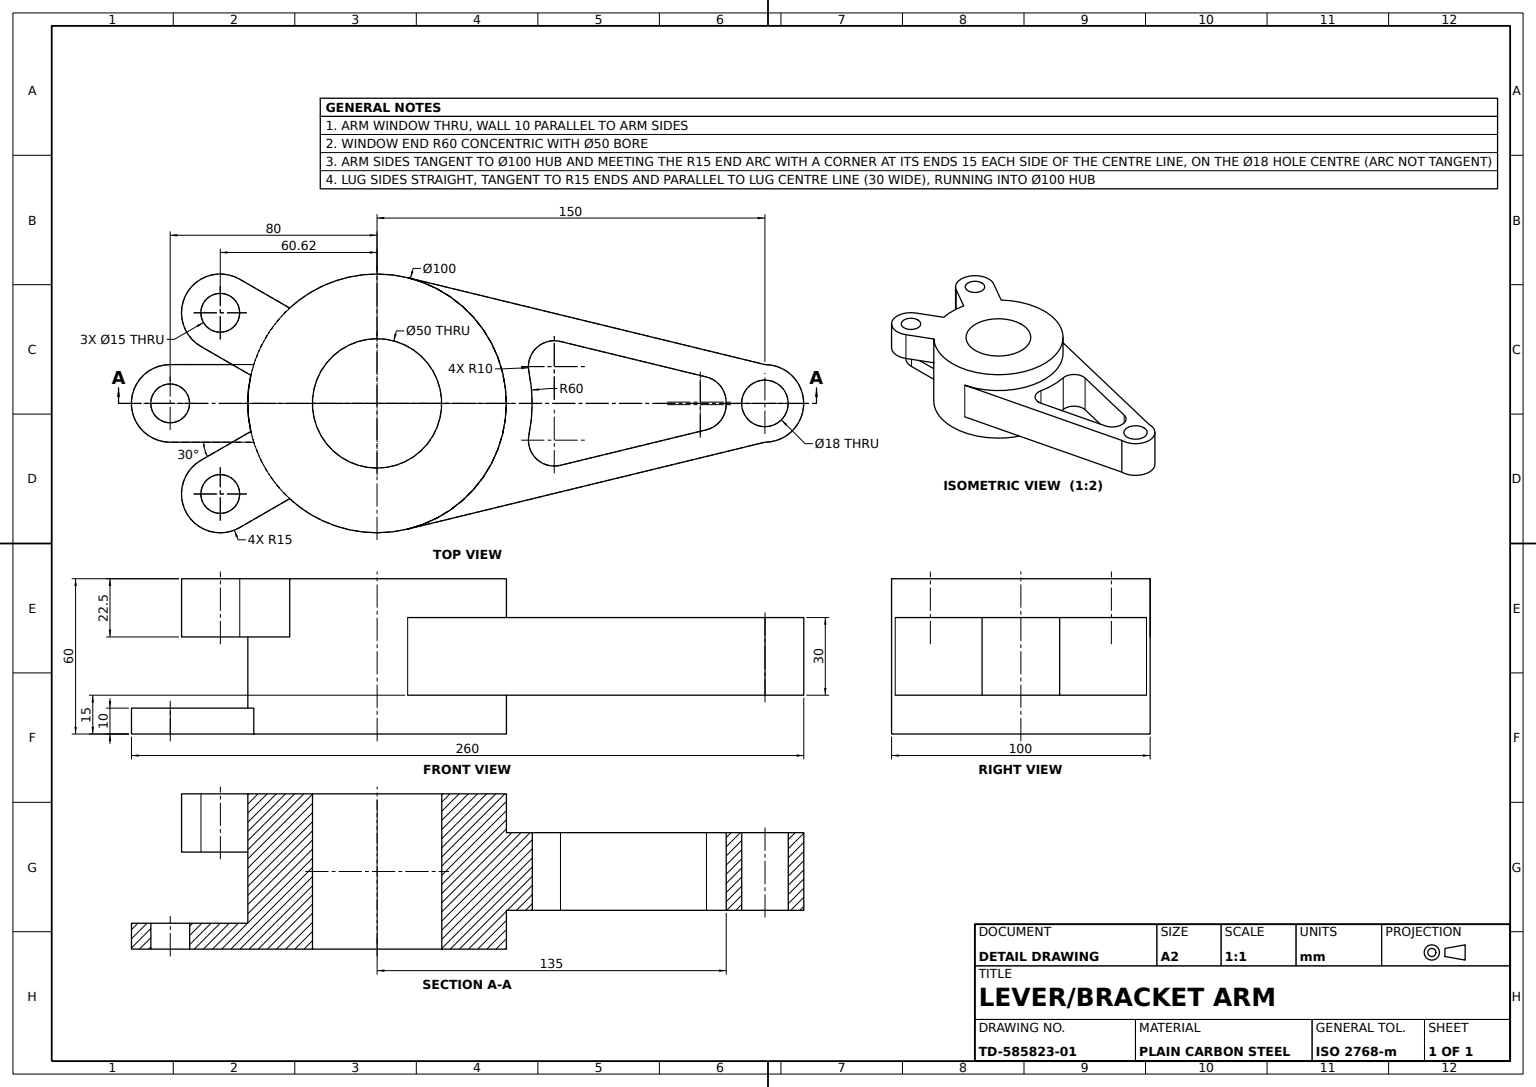
ISO-10303-21;
HEADER;
FILE_DESCRIPTION((''),'2;1');
FILE_NAME('','',(''),(''),'','','');
FILE_SCHEMA(('AUTOMOTIVE_DESIGN'));
ENDSEC;
DATA;
#1=APPLICATION_CONTEXT('');
#2=PRODUCT_CONTEXT('',#1,'mechanical');
#3=PRODUCT('','','',(#2));
#4=PRODUCT_DEFINITION_FORMATION('','',#3);
#5=PRODUCT_DEFINITION_CONTEXT('',#1,'design');
#6=PRODUCT_DEFINITION('','',#4,#5);
#7=PRODUCT_DEFINITION_SHAPE('','',#6);
#8=(LENGTH_UNIT()NAMED_UNIT(*)SI_UNIT(.MILLI.,.METRE.));
#9=(NAMED_UNIT(*)PLANE_ANGLE_UNIT()SI_UNIT($,.RADIAN.));
#10=(NAMED_UNIT(*)SI_UNIT($,.STERADIAN.)SOLID_ANGLE_UNIT());
#11=UNCERTAINTY_MEASURE_WITH_UNIT(LENGTH_MEASURE(1.E-05),#8,'distance_accuracy_value','');
#12=(GEOMETRIC_REPRESENTATION_CONTEXT(3)GLOBAL_UNCERTAINTY_ASSIGNED_CONTEXT((#11))GLOBAL_UNIT_ASSIGNED_CONTEXT((#8,#9,#10))REPRESENTATION_CONTEXT('',''));
#13=CARTESIAN_POINT('',(-53.121778,37.5,-47.990381));
#14=VERTEX_POINT('',#13);
#15=CARTESIAN_POINT('',(-53.121778,60.,-47.990381));
#16=VERTEX_POINT('',#15);
#17=DIRECTION('',(0.,1.,0.));
#18=VECTOR('',#17,1000.);
#19=LINE('',#13,#18);
#20=EDGE_CURVE('',#14,#16,#19,.T.);
#21=ORIENTED_EDGE('',*,*,#20,.T.);
#22=CARTESIAN_POINT('',(-33.806779,60.,-36.838861));
#23=VERTEX_POINT('',#22);
#24=DIRECTION('',(-0.866025404,0.,-0.5));
#25=VECTOR('',#24,1000.);
#26=LINE('',#22,#25);
#27=EDGE_CURVE('',#23,#16,#26,.T.);
#28=ORIENTED_EDGE('',*,*,#27,.F.);
#29=CARTESIAN_POINT('',(-33.806779,37.5,-36.838861));
#30=VERTEX_POINT('',#29);
#31=LINE('',#29,#18);
#32=EDGE_CURVE('',#30,#23,#31,.T.);
#33=ORIENTED_EDGE('',*,*,#32,.F.);
#34=LINE('',#29,#25);
#35=EDGE_CURVE('',#30,#14,#34,.T.);
#36=ORIENTED_EDGE('',*,*,#35,.T.);
#37=EDGE_LOOP('',(#21,#28,#33,#36));
#38=FACE_OUTER_BOUND('',#37,.T.);
#39=DIRECTION('',(0.5,0.,-0.866025404));
#40=AXIS2_PLACEMENT_3D('',#29,#39,#24);
#41=PLANE('',#40);
#42=ADVANCED_FACE('',(#38),#41,.T.);
#43=CARTESIAN_POINT('',(150.,15.,-15.));
#44=VERTEX_POINT('',#43);
#45=CARTESIAN_POINT('',(11.808098,15.,-48.585685));
#46=VERTEX_POINT('',#45);
#47=DIRECTION('',(-0.971713706,0.,-0.236161963));
#48=VECTOR('',#47,1000.);
#49=LINE('',#45,#48);
#50=EDGE_CURVE('',#44,#46,#49,.T.);
#51=ORIENTED_EDGE('',*,*,#50,.T.);
#52=CARTESIAN_POINT('',(11.808098,45.,-48.585685));
#53=VERTEX_POINT('',#52);
#54=DIRECTION('',(0.,-1.,0.));
#55=VECTOR('',#54,1000.);
#56=LINE('',#52,#55);
#57=EDGE_CURVE('',#53,#46,#56,.T.);
#58=ORIENTED_EDGE('',*,*,#57,.F.);
#59=CARTESIAN_POINT('',(150.,45.,-15.));
#60=VERTEX_POINT('',#59);
#61=LINE('',#52,#48);
#62=EDGE_CURVE('',#60,#53,#61,.T.);
#63=ORIENTED_EDGE('',*,*,#62,.F.);
#64=LINE('',#59,#55);
#65=EDGE_CURVE('',#60,#44,#64,.T.);
#66=ORIENTED_EDGE('',*,*,#65,.T.);
#67=EDGE_LOOP('',(#51,#58,#63,#66));
#68=FACE_OUTER_BOUND('',#67,.T.);
#69=DIRECTION('',(-0.236161963,0.,0.971713706));
#70=DIRECTION('',(0.971713706,0.,0.236161963));
#71=AXIS2_PLACEMENT_3D('',#52,#69,#70);
#72=PLANE('',#71);
#73=ADVANCED_FACE('',(#68),#72,.F.);
#74=CARTESIAN_POINT('',(0.,60.,-25.));
#75=VERTEX_POINT('',#74);
#76=CARTESIAN_POINT('',(0.,0.,-25.));
#77=VERTEX_POINT('',#76);
#78=LINE('',#74,#55);
#79=EDGE_CURVE('',#75,#77,#78,.T.);
#80=ORIENTED_EDGE('',*,*,#79,.T.);
#81=CARTESIAN_POINT('',(0.,0.,25.));
#82=VERTEX_POINT('',#81);
#83=CARTESIAN_POINT('',(0.,0.,0.));
#84=DIRECTION('',(0.,0.,1.));
#85=AXIS2_PLACEMENT_3D('',#83,#17,#84);
#86=CIRCLE('',#85,25.);
#87=EDGE_CURVE('',#82,#77,#86,.T.);
#88=ORIENTED_EDGE('',*,*,#87,.F.);
#89=CARTESIAN_POINT('',(0.,60.,25.));
#90=VERTEX_POINT('',#89);
#91=LINE('',#89,#55);
#92=EDGE_CURVE('',#90,#82,#91,.T.);
#93=ORIENTED_EDGE('',*,*,#92,.F.);
#94=CARTESIAN_POINT('',(0.,60.,0.));
#95=AXIS2_PLACEMENT_3D('',#94,#17,#84);
#96=CIRCLE('',#95,25.);
#97=EDGE_CURVE('',#90,#75,#96,.T.);
#98=ORIENTED_EDGE('',*,*,#97,.T.);
#99=EDGE_LOOP('',(#80,#88,#93,#98));
#100=FACE_OUTER_BOUND('',#99,.T.);
#101=DIRECTION('',(0.,0.,-1.));
#102=AXIS2_PLACEMENT_3D('',#94,#54,#101);
#103=CYLINDRICAL_SURFACE('',#102,25.);
#104=ADVANCED_FACE('',(#100),#103,.F.);
#105=CARTESIAN_POINT('',(-68.121778,37.5,22.009619));
#106=VERTEX_POINT('',#105);
#107=CARTESIAN_POINT('',(-60.621778,37.5,50.));
#108=VERTEX_POINT('',#107);
#109=CARTESIAN_POINT('',(-60.621778,37.5,35.));
#110=AXIS2_PLACEMENT_3D('',#109,#17,#84);
#111=CIRCLE('',#110,15.);
#112=EDGE_CURVE('',#106,#108,#111,.T.);
#113=ORIENTED_EDGE('',*,*,#112,.T.);
#114=CARTESIAN_POINT('',(-60.621778,60.,50.));
#115=VERTEX_POINT('',#114);
#116=LINE('',#107,#18);
#117=EDGE_CURVE('',#108,#115,#116,.T.);
#118=ORIENTED_EDGE('',*,*,#117,.T.);
#119=CARTESIAN_POINT('',(-68.121778,60.,22.009619));
#120=VERTEX_POINT('',#119);
#121=CARTESIAN_POINT('',(-60.621778,60.,35.));
#122=AXIS2_PLACEMENT_3D('',#121,#17,#84);
#123=CIRCLE('',#122,15.);
#124=EDGE_CURVE('',#120,#115,#123,.T.);
#125=ORIENTED_EDGE('',*,*,#124,.F.);
#126=LINE('',#105,#18);
#127=EDGE_CURVE('',#106,#120,#126,.T.);
#128=ORIENTED_EDGE('',*,*,#127,.F.);
#129=EDGE_LOOP('',(#113,#118,#125,#128));
#130=FACE_OUTER_BOUND('',#129,.T.);
#131=CYLINDRICAL_SURFACE('',#110,15.);
#132=ADVANCED_FACE('',(#130),#131,.T.);
#133=CARTESIAN_POINT('',(-60.621778,37.5,27.5));
#134=VERTEX_POINT('',#133);
#135=CARTESIAN_POINT('',(-60.621778,37.5,42.5));
#136=VERTEX_POINT('',#135);
#137=CIRCLE('',#110,7.5);
#138=EDGE_CURVE('',#134,#136,#137,.T.);
#139=ORIENTED_EDGE('',*,*,#138,.T.);
#140=EDGE_CURVE('',#136,#134,#137,.T.);
#141=ORIENTED_EDGE('',*,*,#140,.T.);
#142=EDGE_LOOP('',(#139,#141));
#143=FACE_BOUND('',#142,.T.);
#144=ORIENTED_EDGE('',*,*,#112,.F.);
#145=CARTESIAN_POINT('',(-48.806779,37.5,10.858099));
#146=VERTEX_POINT('',#145);
#147=CARTESIAN_POINT('',(-48.770061,37.5,10.8369));
#148=DIRECTION('',(-0.866025404,0.,0.5));
#149=VECTOR('',#148,1000.);
#150=LINE('',#147,#149);
#151=EDGE_CURVE('',#146,#106,#150,.T.);
#152=ORIENTED_EDGE('',*,*,#151,.F.);
#153=CARTESIAN_POINT('',(-33.806779,37.5,36.838861));
#154=VERTEX_POINT('',#153);
#155=CARTESIAN_POINT('',(0.,37.5,0.));
#156=AXIS2_PLACEMENT_3D('',#155,#17,#84);
#157=CIRCLE('',#156,50.);
#158=EDGE_CURVE('',#146,#154,#157,.T.);
#159=ORIENTED_EDGE('',*,*,#158,.T.);
#160=CARTESIAN_POINT('',(-53.121778,37.5,47.990381));
#161=VERTEX_POINT('',#160);
#162=CARTESIAN_POINT('',(-33.644954,37.5,36.745431));
#163=DIRECTION('',(0.866025404,0.,-0.5));
#164=VECTOR('',#163,1000.);
#165=LINE('',#162,#164);
#166=EDGE_CURVE('',#161,#154,#165,.T.);
#167=ORIENTED_EDGE('',*,*,#166,.F.);
#168=EDGE_CURVE('',#108,#161,#111,.T.);
#169=ORIENTED_EDGE('',*,*,#168,.F.);
#170=EDGE_LOOP('',(#144,#152,#159,#167,#169));
#171=FACE_OUTER_BOUND('',#170,.T.);
#172=PLANE('',#110);
#173=ADVANCED_FACE('',(#143,#171),#172,.F.);
#174=CARTESIAN_POINT('',(127.366472,15.,-10.209678));
#175=VERTEX_POINT('',#174);
#176=CARTESIAN_POINT('',(135.002911,15.,-0.295525));
#177=VERTEX_POINT('',#176);
#178=CARTESIAN_POINT('',(125.004852,15.,-0.492541));
#179=AXIS2_PLACEMENT_3D('',#178,#54,#101);
#180=CIRCLE('',#179,10.);
#181=EDGE_CURVE('',#175,#177,#180,.T.);
#182=ORIENTED_EDGE('',*,*,#181,.T.);
#183=CARTESIAN_POINT('',(135.002911,45.,-0.295525));
#184=VERTEX_POINT('',#183);
#185=CARTESIAN_POINT('',(135.002911,0.,-0.295525));
#186=LINE('',#185,#18);
#187=EDGE_CURVE('',#177,#184,#186,.T.);
#188=ORIENTED_EDGE('',*,*,#187,.T.);
#189=CARTESIAN_POINT('',(127.366472,45.,-10.209678));
#190=VERTEX_POINT('',#189);
#191=CARTESIAN_POINT('',(125.004852,45.,-0.492541));
#192=AXIS2_PLACEMENT_3D('',#191,#17,#84);
#193=CIRCLE('',#192,10.);
#194=EDGE_CURVE('',#184,#190,#193,.T.);
#195=ORIENTED_EDGE('',*,*,#194,.T.);
#196=CARTESIAN_POINT('',(127.366472,0.,-10.209678));
#197=LINE('',#196,#18);
#198=EDGE_CURVE('',#175,#190,#197,.T.);
#199=ORIENTED_EDGE('',*,*,#198,.F.);
#200=EDGE_LOOP('',(#182,#188,#195,#199));
#201=FACE_OUTER_BOUND('',#200,.T.);
#202=CARTESIAN_POINT('',(125.004852,0.,-0.492541));
#203=AXIS2_PLACEMENT_3D('',#202,#17,#84);
#204=CYLINDRICAL_SURFACE('',#203,10.);
#205=ADVANCED_FACE('',(#201),#204,.F.);
#206=CARTESIAN_POINT('',(-80.,0.,-7.5));
#207=VERTEX_POINT('',#206);
#208=CARTESIAN_POINT('',(-80.,0.,7.5));
#209=VERTEX_POINT('',#208);
#210=CARTESIAN_POINT('',(-80.,0.,0.));
#211=AXIS2_PLACEMENT_3D('',#210,#17,#84);
#212=CIRCLE('',#211,7.5);
#213=EDGE_CURVE('',#207,#209,#212,.T.);
#214=ORIENTED_EDGE('',*,*,#213,.T.);
#215=EDGE_CURVE('',#209,#207,#212,.T.);
#216=ORIENTED_EDGE('',*,*,#215,.T.);
#217=EDGE_LOOP('',(#214,#216));
#218=FACE_BOUND('',#217,.T.);
#219=CARTESIAN_POINT('',(-47.69696,0.,15.));
#220=VERTEX_POINT('',#219);
#221=CARTESIAN_POINT('',(0.,0.,50.));
#222=VERTEX_POINT('',#221);
#223=CIRCLE('',#85,50.);
#224=EDGE_CURVE('',#220,#222,#223,.T.);
#225=ORIENTED_EDGE('',*,*,#224,.F.);
#226=CARTESIAN_POINT('',(-80.,0.,15.));
#227=VERTEX_POINT('',#226);
#228=DIRECTION('',(1.,0.,0.));
#229=VECTOR('',#228,1000.);
#230=LINE('',#226,#229);
#231=EDGE_CURVE('',#227,#220,#230,.T.);
#232=ORIENTED_EDGE('',*,*,#231,.F.);
#233=CARTESIAN_POINT('',(-80.,0.,-15.));
#234=VERTEX_POINT('',#233);
#235=CIRCLE('',#211,15.);
#236=EDGE_CURVE('',#234,#227,#235,.T.);
#237=ORIENTED_EDGE('',*,*,#236,.F.);
#238=CARTESIAN_POINT('',(-47.69696,0.,-15.));
#239=VERTEX_POINT('',#238);
#240=DIRECTION('',(-1.,0.,0.));
#241=VECTOR('',#240,1000.);
#242=LINE('',#233,#241);
#243=EDGE_CURVE('',#239,#234,#242,.T.);
#244=ORIENTED_EDGE('',*,*,#243,.F.);
#245=CARTESIAN_POINT('',(0.,0.,-50.));
#246=VERTEX_POINT('',#245);
#247=EDGE_CURVE('',#246,#239,#223,.T.);
#248=ORIENTED_EDGE('',*,*,#247,.F.);
#249=EDGE_CURVE('',#222,#246,#223,.T.);
#250=ORIENTED_EDGE('',*,*,#249,.F.);
#251=EDGE_LOOP('',(#225,#232,#237,#244,#248,#250));
#252=FACE_OUTER_BOUND('',#251,.T.);
#253=EDGE_CURVE('',#77,#82,#86,.T.);
#254=ORIENTED_EDGE('',*,*,#253,.T.);
#255=ORIENTED_EDGE('',*,*,#87,.T.);
#256=EDGE_LOOP('',(#254,#255));
#257=FACE_BOUND('',#256,.T.);
#258=PLANE('',#85);
#259=ADVANCED_FACE('',(#218,#252,#257),#258,.F.);
#260=EDGE_CURVE('',#75,#90,#96,.T.);
#261=ORIENTED_EDGE('',*,*,#260,.T.);
#262=ORIENTED_EDGE('',*,*,#92,.T.);
#263=ORIENTED_EDGE('',*,*,#253,.F.);
#264=ORIENTED_EDGE('',*,*,#79,.F.);
#265=EDGE_LOOP('',(#261,#262,#263,#264));
#266=FACE_OUTER_BOUND('',#265,.T.);
#267=ADVANCED_FACE('',(#266),#103,.F.);
#268=CARTESIAN_POINT('',(-33.806779,60.,36.838861));
#269=VERTEX_POINT('',#268);
#270=LINE('',#268,#55);
#271=EDGE_CURVE('',#269,#154,#270,.T.);
#272=ORIENTED_EDGE('',*,*,#271,.F.);
#273=CARTESIAN_POINT('',(-53.121778,60.,47.990381));
#274=VERTEX_POINT('',#273);
#275=CARTESIAN_POINT('',(-33.644954,60.,36.745431));
#276=LINE('',#275,#164);
#277=EDGE_CURVE('',#274,#269,#276,.T.);
#278=ORIENTED_EDGE('',*,*,#277,.F.);
#279=LINE('',#160,#18);
#280=EDGE_CURVE('',#161,#274,#279,.T.);
#281=ORIENTED_EDGE('',*,*,#280,.F.);
#282=ORIENTED_EDGE('',*,*,#166,.T.);
#283=EDGE_LOOP('',(#272,#278,#281,#282));
#284=FACE_OUTER_BOUND('',#283,.T.);
#285=DIRECTION('',(0.5,0.,0.866025404));
#286=AXIS2_PLACEMENT_3D('',#162,#285,#163);
#287=PLANE('',#286);
#288=ADVANCED_FACE('',(#284),#287,.T.);
#289=CARTESIAN_POINT('',(150.,45.,15.));
#290=VERTEX_POINT('',#289);
#291=CARTESIAN_POINT('',(150.,15.,15.));
#292=VERTEX_POINT('',#291);
#293=LINE('',#289,#55);
#294=EDGE_CURVE('',#290,#292,#293,.T.);
#295=ORIENTED_EDGE('',*,*,#294,.F.);
#296=CARTESIAN_POINT('',(11.808098,45.,48.585685));
#297=VERTEX_POINT('',#296);
#298=DIRECTION('',(0.971713706,0.,-0.236161963));
#299=VECTOR('',#298,1000.);
#300=LINE('',#296,#299);
#301=EDGE_CURVE('',#297,#290,#300,.T.);
#302=ORIENTED_EDGE('',*,*,#301,.F.);
#303=CARTESIAN_POINT('',(11.808098,15.,48.585685));
#304=VERTEX_POINT('',#303);
#305=LINE('',#296,#55);
#306=EDGE_CURVE('',#297,#304,#305,.T.);
#307=ORIENTED_EDGE('',*,*,#306,.T.);
#308=LINE('',#303,#299);
#309=EDGE_CURVE('',#304,#292,#308,.T.);
#310=ORIENTED_EDGE('',*,*,#309,.T.);
#311=EDGE_LOOP('',(#295,#302,#307,#310));
#312=FACE_OUTER_BOUND('',#311,.T.);
#313=DIRECTION('',(-0.236161963,0.,-0.971713706));
#314=DIRECTION('',(-0.971713706,0.,0.236161963));
#315=AXIS2_PLACEMENT_3D('',#296,#313,#314);
#316=PLANE('',#315);
#317=ADVANCED_FACE('',(#312),#316,.F.);
#318=ORIENTED_EDGE('',*,*,#236,.T.);
#319=CARTESIAN_POINT('',(-80.,10.,15.));
#320=VERTEX_POINT('',#319);
#321=LINE('',#319,#55);
#322=EDGE_CURVE('',#320,#227,#321,.T.);
#323=ORIENTED_EDGE('',*,*,#322,.F.);
#324=CARTESIAN_POINT('',(-80.,10.,-15.));
#325=VERTEX_POINT('',#324);
#326=CARTESIAN_POINT('',(-80.,10.,0.));
#327=AXIS2_PLACEMENT_3D('',#326,#17,#84);
#328=CIRCLE('',#327,15.);
#329=EDGE_CURVE('',#325,#320,#328,.T.);
#330=ORIENTED_EDGE('',*,*,#329,.F.);
#331=LINE('',#324,#55);
#332=EDGE_CURVE('',#325,#234,#331,.T.);
#333=ORIENTED_EDGE('',*,*,#332,.T.);
#334=EDGE_LOOP('',(#318,#323,#330,#333));
#335=FACE_OUTER_BOUND('',#334,.T.);
#336=AXIS2_PLACEMENT_3D('',#326,#54,#101);
#337=CYLINDRICAL_SURFACE('',#336,15.);
#338=ADVANCED_FACE('',(#335),#337,.T.);
#339=CARTESIAN_POINT('',(-48.806779,60.,10.858099));
#340=VERTEX_POINT('',#339);
#341=LINE('',#339,#18);
#342=EDGE_CURVE('',#146,#340,#341,.T.);
#343=ORIENTED_EDGE('',*,*,#342,.T.);
#344=CARTESIAN_POINT('',(-48.806779,60.,-10.858099));
#345=VERTEX_POINT('',#344);
#346=CIRCLE('',#95,50.);
#347=EDGE_CURVE('',#345,#340,#346,.T.);
#348=ORIENTED_EDGE('',*,*,#347,.F.);
#349=CARTESIAN_POINT('',(-48.806779,37.5,-10.858099));
#350=VERTEX_POINT('',#349);
#351=LINE('',#349,#18);
#352=EDGE_CURVE('',#350,#345,#351,.T.);
#353=ORIENTED_EDGE('',*,*,#352,.F.);
#354=AXIS2_PLACEMENT_3D('',#155,#54,#84);
#355=CIRCLE('',#354,50.);
#356=EDGE_CURVE('',#350,#30,#355,.T.);
#357=ORIENTED_EDGE('',*,*,#356,.T.);
#358=ORIENTED_EDGE('',*,*,#32,.T.);
#359=CARTESIAN_POINT('',(0.,60.,-50.));
#360=VERTEX_POINT('',#359);
#361=EDGE_CURVE('',#360,#23,#346,.T.);
#362=ORIENTED_EDGE('',*,*,#361,.F.);
#363=LINE('',#359,#55);
#364=EDGE_CURVE('',#360,#246,#363,.T.);
#365=ORIENTED_EDGE('',*,*,#364,.T.);
#366=ORIENTED_EDGE('',*,*,#247,.T.);
#367=CARTESIAN_POINT('',(-47.69696,10.,-15.));
#368=VERTEX_POINT('',#367);
#369=CARTESIAN_POINT('',(-47.69696,60.,-15.));
#370=LINE('',#369,#55);
#371=EDGE_CURVE('',#368,#239,#370,.T.);
#372=ORIENTED_EDGE('',*,*,#371,.F.);
#373=CARTESIAN_POINT('',(-47.69696,10.,15.));
#374=VERTEX_POINT('',#373);
#375=CARTESIAN_POINT('',(0.,10.,0.));
#376=AXIS2_PLACEMENT_3D('',#375,#17,#84);
#377=CIRCLE('',#376,50.);
#378=EDGE_CURVE('',#368,#374,#377,.T.);
#379=ORIENTED_EDGE('',*,*,#378,.T.);
#380=CARTESIAN_POINT('',(-47.69696,60.,15.));
#381=LINE('',#380,#18);
#382=EDGE_CURVE('',#220,#374,#381,.T.);
#383=ORIENTED_EDGE('',*,*,#382,.F.);
#384=ORIENTED_EDGE('',*,*,#224,.T.);
#385=CARTESIAN_POINT('',(0.,60.,50.));
#386=VERTEX_POINT('',#385);
#387=LINE('',#385,#55);
#388=EDGE_CURVE('',#386,#222,#387,.T.);
#389=ORIENTED_EDGE('',*,*,#388,.F.);
#390=EDGE_CURVE('',#269,#386,#346,.T.);
#391=ORIENTED_EDGE('',*,*,#390,.F.);
#392=ORIENTED_EDGE('',*,*,#271,.T.);
#393=ORIENTED_EDGE('',*,*,#158,.F.);
#394=EDGE_LOOP('',(#343,#348,#353,#357,#358,#362,#365,#366,#372,#379,#383,#384,#389,#391,#392,#393));
#395=FACE_OUTER_BOUND('',#394,.T.);
#396=CYLINDRICAL_SURFACE('',#102,50.);
#397=ADVANCED_FACE('',(#395),#396,.T.);
#398=CARTESIAN_POINT('',(70.903049,15.,23.932354));
#399=VERTEX_POINT('',#398);
#400=CARTESIAN_POINT('',(70.903049,45.,23.932354));
#401=VERTEX_POINT('',#400);
#402=CARTESIAN_POINT('',(70.903049,0.,23.932354));
#403=LINE('',#402,#18);
#404=EDGE_CURVE('',#399,#401,#403,.T.);
#405=ORIENTED_EDGE('',*,*,#404,.F.);
#406=CARTESIAN_POINT('',(68.54143,15.,24.215217));
#407=VERTEX_POINT('',#406);
#408=CARTESIAN_POINT('',(68.54143,15.,14.215217));
#409=AXIS2_PLACEMENT_3D('',#408,#54,#101);
#410=CIRCLE('',#409,10.);
#411=EDGE_CURVE('',#399,#407,#410,.T.);
#412=ORIENTED_EDGE('',*,*,#411,.T.);
#413=CARTESIAN_POINT('',(68.54143,45.,24.215217));
#414=VERTEX_POINT('',#413);
#415=CARTESIAN_POINT('',(68.54143,0.,24.215217));
#416=LINE('',#415,#18);
#417=EDGE_CURVE('',#407,#414,#416,.T.);
#418=ORIENTED_EDGE('',*,*,#417,.T.);
#419=CARTESIAN_POINT('',(68.54143,45.,14.215217));
#420=AXIS2_PLACEMENT_3D('',#419,#17,#84);
#421=CIRCLE('',#420,10.);
#422=EDGE_CURVE('',#414,#401,#421,.T.);
#423=ORIENTED_EDGE('',*,*,#422,.T.);
#424=EDGE_LOOP('',(#405,#412,#418,#423));
#425=FACE_OUTER_BOUND('',#424,.T.);
#426=CARTESIAN_POINT('',(68.54143,0.,14.215217));
#427=AXIS2_PLACEMENT_3D('',#426,#17,#84);
#428=CYLINDRICAL_SURFACE('',#427,10.);
#429=ADVANCED_FACE('',(#425),#428,.F.);
#430=ORIENTED_EDGE('',*,*,#404,.T.);
#431=CARTESIAN_POINT('',(127.366472,45.,10.209678));
#432=VERTEX_POINT('',#431);
#433=LINE('',#400,#299);
#434=EDGE_CURVE('',#401,#432,#433,.T.);
#435=ORIENTED_EDGE('',*,*,#434,.T.);
#436=CARTESIAN_POINT('',(127.366472,15.,10.209678));
#437=VERTEX_POINT('',#436);
#438=CARTESIAN_POINT('',(127.366472,0.,10.209678));
#439=LINE('',#438,#18);
#440=EDGE_CURVE('',#437,#432,#439,.T.);
#441=ORIENTED_EDGE('',*,*,#440,.F.);
#442=CARTESIAN_POINT('',(9.446479,15.,38.868548));
#443=VECTOR('',#314,1000.);
#444=LINE('',#442,#443);
#445=EDGE_CURVE('',#437,#399,#444,.T.);
#446=ORIENTED_EDGE('',*,*,#445,.T.);
#447=EDGE_LOOP('',(#430,#435,#441,#446));
#448=FACE_OUTER_BOUND('',#447,.T.);
#449=DIRECTION('',(0.236161963,0.,0.971713706));
#450=AXIS2_PLACEMENT_3D('',#402,#449,#298);
#451=PLANE('',#450);
#452=ADVANCED_FACE('',(#448),#451,.F.);
#453=CARTESIAN_POINT('',(58.749797,15.,12.184472));
#454=VERTEX_POINT('',#453);
#455=CARTESIAN_POINT('',(58.749797,15.,-12.184472));
#456=VERTEX_POINT('',#455);
#457=CARTESIAN_POINT('',(0.,15.,0.));
#458=AXIS2_PLACEMENT_3D('',#457,#17,#101);
#459=CIRCLE('',#458,60.);
#460=EDGE_CURVE('',#454,#456,#459,.T.);
#461=ORIENTED_EDGE('',*,*,#460,.T.);
#462=CARTESIAN_POINT('',(58.749797,45.,-12.184472));
#463=VERTEX_POINT('',#462);
#464=CARTESIAN_POINT('',(58.749797,0.,-12.184472));
#465=LINE('',#464,#18);
#466=EDGE_CURVE('',#456,#463,#465,.T.);
#467=ORIENTED_EDGE('',*,*,#466,.T.);
#468=CARTESIAN_POINT('',(58.749797,45.,12.184472));
#469=VERTEX_POINT('',#468);
#470=CARTESIAN_POINT('',(0.,45.,0.));
#471=AXIS2_PLACEMENT_3D('',#470,#54,#84);
#472=CIRCLE('',#471,60.);
#473=EDGE_CURVE('',#463,#469,#472,.T.);
#474=ORIENTED_EDGE('',*,*,#473,.T.);
#475=CARTESIAN_POINT('',(58.749797,0.,12.184472));
#476=LINE('',#475,#18);
#477=EDGE_CURVE('',#454,#469,#476,.T.);
#478=ORIENTED_EDGE('',*,*,#477,.F.);
#479=EDGE_LOOP('',(#461,#467,#474,#478));
#480=FACE_OUTER_BOUND('',#479,.T.);
#481=CYLINDRICAL_SURFACE('',#85,60.);
#482=ADVANCED_FACE('',(#480),#481,.T.);
#483=CARTESIAN_POINT('',(-60.621778,60.,42.5));
#484=VERTEX_POINT('',#483);
#485=LINE('',#135,#18);
#486=EDGE_CURVE('',#136,#484,#485,.T.);
#487=ORIENTED_EDGE('',*,*,#486,.T.);
#488=CARTESIAN_POINT('',(-60.621778,60.,27.5));
#489=VERTEX_POINT('',#488);
#490=CIRCLE('',#122,7.5);
#491=EDGE_CURVE('',#484,#489,#490,.T.);
#492=ORIENTED_EDGE('',*,*,#491,.T.);
#493=LINE('',#133,#18);
#494=EDGE_CURVE('',#134,#489,#493,.T.);
#495=ORIENTED_EDGE('',*,*,#494,.F.);
#496=ORIENTED_EDGE('',*,*,#140,.F.);
#497=EDGE_LOOP('',(#487,#492,#495,#496));
#498=FACE_OUTER_BOUND('',#497,.T.);
#499=CYLINDRICAL_SURFACE('',#110,7.5);
#500=ADVANCED_FACE('',(#498),#499,.F.);
#501=CARTESIAN_POINT('',(-60.621778,60.,-27.5));
#502=VERTEX_POINT('',#501);
#503=CARTESIAN_POINT('',(-60.621778,60.,-42.5));
#504=VERTEX_POINT('',#503);
#505=CARTESIAN_POINT('',(-60.621778,60.,-35.));
#506=AXIS2_PLACEMENT_3D('',#505,#17,#84);
#507=CIRCLE('',#506,7.5);
#508=EDGE_CURVE('',#502,#504,#507,.T.);
#509=ORIENTED_EDGE('',*,*,#508,.T.);
#510=CARTESIAN_POINT('',(-60.621778,37.5,-42.5));
#511=VERTEX_POINT('',#510);
#512=LINE('',#510,#18);
#513=EDGE_CURVE('',#511,#504,#512,.T.);
#514=ORIENTED_EDGE('',*,*,#513,.F.);
#515=CARTESIAN_POINT('',(-60.621778,37.5,-27.5));
#516=VERTEX_POINT('',#515);
#517=CARTESIAN_POINT('',(-60.621778,37.5,-35.));
#518=AXIS2_PLACEMENT_3D('',#517,#17,#84);
#519=CIRCLE('',#518,7.5);
#520=EDGE_CURVE('',#516,#511,#519,.T.);
#521=ORIENTED_EDGE('',*,*,#520,.F.);
#522=LINE('',#515,#18);
#523=EDGE_CURVE('',#516,#502,#522,.T.);
#524=ORIENTED_EDGE('',*,*,#523,.T.);
#525=EDGE_LOOP('',(#509,#514,#521,#524));
#526=FACE_OUTER_BOUND('',#525,.T.);
#527=CYLINDRICAL_SURFACE('',#518,7.5);
#528=ADVANCED_FACE('',(#526),#527,.F.);
#529=CARTESIAN_POINT('',(-68.121778,37.5,-22.009619));
#530=VERTEX_POINT('',#529);
#531=CIRCLE('',#518,15.);
#532=EDGE_CURVE('',#14,#530,#531,.T.);
#533=ORIENTED_EDGE('',*,*,#532,.T.);
#534=CARTESIAN_POINT('',(-68.121778,60.,-22.009619));
#535=VERTEX_POINT('',#534);
#536=LINE('',#529,#18);
#537=EDGE_CURVE('',#530,#535,#536,.T.);
#538=ORIENTED_EDGE('',*,*,#537,.T.);
#539=CIRCLE('',#506,15.);
#540=EDGE_CURVE('',#16,#535,#539,.T.);
#541=ORIENTED_EDGE('',*,*,#540,.F.);
#542=ORIENTED_EDGE('',*,*,#20,.F.);
#543=EDGE_LOOP('',(#533,#538,#541,#542));
#544=FACE_OUTER_BOUND('',#543,.T.);
#545=CYLINDRICAL_SURFACE('',#518,15.);
#546=ADVANCED_FACE('',(#544),#545,.T.);
#547=CARTESIAN_POINT('',(150.,45.,9.));
#548=VERTEX_POINT('',#547);
#549=CARTESIAN_POINT('',(150.,45.,-9.));
#550=VERTEX_POINT('',#549);
#551=CARTESIAN_POINT('',(150.,45.,0.));
#552=AXIS2_PLACEMENT_3D('',#551,#17,#84);
#553=CIRCLE('',#552,9.);
#554=EDGE_CURVE('',#548,#550,#553,.T.);
#555=ORIENTED_EDGE('',*,*,#554,.T.);
#556=CARTESIAN_POINT('',(150.,15.,-9.));
#557=VERTEX_POINT('',#556);
#558=LINE('',#549,#55);
#559=EDGE_CURVE('',#550,#557,#558,.T.);
#560=ORIENTED_EDGE('',*,*,#559,.T.);
#561=CARTESIAN_POINT('',(150.,15.,9.));
#562=VERTEX_POINT('',#561);
#563=CARTESIAN_POINT('',(150.,15.,0.));
#564=AXIS2_PLACEMENT_3D('',#563,#17,#84);
#565=CIRCLE('',#564,9.);
#566=EDGE_CURVE('',#562,#557,#565,.T.);
#567=ORIENTED_EDGE('',*,*,#566,.F.);
#568=LINE('',#547,#55);
#569=EDGE_CURVE('',#548,#562,#568,.T.);
#570=ORIENTED_EDGE('',*,*,#569,.F.);
#571=EDGE_LOOP('',(#555,#560,#567,#570));
#572=FACE_OUTER_BOUND('',#571,.T.);
#573=AXIS2_PLACEMENT_3D('',#551,#54,#101);
#574=CYLINDRICAL_SURFACE('',#573,9.);
#575=ADVANCED_FACE('',(#572),#574,.F.);
#576=CIRCLE('',#552,15.);
#577=EDGE_CURVE('',#290,#60,#576,.T.);
#578=ORIENTED_EDGE('',*,*,#577,.F.);
#579=ORIENTED_EDGE('',*,*,#294,.T.);
#580=CIRCLE('',#564,15.);
#581=EDGE_CURVE('',#292,#44,#580,.T.);
#582=ORIENTED_EDGE('',*,*,#581,.T.);
#583=ORIENTED_EDGE('',*,*,#65,.F.);
#584=EDGE_LOOP('',(#578,#579,#582,#583));
#585=FACE_OUTER_BOUND('',#584,.T.);
#586=CYLINDRICAL_SURFACE('',#573,15.);
#587=ADVANCED_FACE('',(#585),#586,.T.);
#588=ORIENTED_EDGE('',*,*,#280,.T.);
#589=EDGE_CURVE('',#115,#274,#123,.T.);
#590=ORIENTED_EDGE('',*,*,#589,.F.);
#591=ORIENTED_EDGE('',*,*,#117,.F.);
#592=ORIENTED_EDGE('',*,*,#168,.T.);
#593=EDGE_LOOP('',(#588,#590,#591,#592));
#594=FACE_OUTER_BOUND('',#593,.T.);
#595=ADVANCED_FACE('',(#594),#131,.T.);
#596=ORIENTED_EDGE('',*,*,#213,.F.);
#597=CARTESIAN_POINT('',(-80.,10.,-7.5));
#598=VERTEX_POINT('',#597);
#599=LINE('',#597,#55);
#600=EDGE_CURVE('',#598,#207,#599,.T.);
#601=ORIENTED_EDGE('',*,*,#600,.F.);
#602=CARTESIAN_POINT('',(-80.,10.,7.5));
#603=VERTEX_POINT('',#602);
#604=CIRCLE('',#327,7.5);
#605=EDGE_CURVE('',#598,#603,#604,.T.);
#606=ORIENTED_EDGE('',*,*,#605,.T.);
#607=LINE('',#602,#55);
#608=EDGE_CURVE('',#603,#209,#607,.T.);
#609=ORIENTED_EDGE('',*,*,#608,.T.);
#610=EDGE_LOOP('',(#596,#601,#606,#609));
#611=FACE_OUTER_BOUND('',#610,.T.);
#612=CYLINDRICAL_SURFACE('',#336,7.5);
#613=ADVANCED_FACE('',(#611),#612,.F.);
#614=CARTESIAN_POINT('',(70.903049,15.,-23.932354));
#615=VERTEX_POINT('',#614);
#616=CARTESIAN_POINT('',(9.446479,15.,-38.868548));
#617=VECTOR('',#70,1000.);
#618=LINE('',#616,#617);
#619=EDGE_CURVE('',#615,#175,#618,.T.);
#620=ORIENTED_EDGE('',*,*,#619,.T.);
#621=ORIENTED_EDGE('',*,*,#198,.T.);
#622=CARTESIAN_POINT('',(70.903049,45.,-23.932354));
#623=VERTEX_POINT('',#622);
#624=LINE('',#189,#48);
#625=EDGE_CURVE('',#190,#623,#624,.T.);
#626=ORIENTED_EDGE('',*,*,#625,.T.);
#627=CARTESIAN_POINT('',(70.903049,0.,-23.932354));
#628=LINE('',#627,#18);
#629=EDGE_CURVE('',#615,#623,#628,.T.);
#630=ORIENTED_EDGE('',*,*,#629,.F.);
#631=EDGE_LOOP('',(#620,#621,#626,#630));
#632=FACE_OUTER_BOUND('',#631,.T.);
#633=DIRECTION('',(0.236161963,0.,-0.971713706));
#634=AXIS2_PLACEMENT_3D('',#196,#633,#47);
#635=PLANE('',#634);
#636=ADVANCED_FACE('',(#632),#635,.F.);
#637=ORIENTED_EDGE('',*,*,#35,.F.);
#638=ORIENTED_EDGE('',*,*,#356,.F.);
#639=DIRECTION('',(0.866025404,0.,0.5));
#640=VECTOR('',#639,1000.);
#641=LINE('',#349,#640);
#642=EDGE_CURVE('',#530,#350,#641,.T.);
#643=ORIENTED_EDGE('',*,*,#642,.F.);
#644=ORIENTED_EDGE('',*,*,#532,.F.);
#645=EDGE_LOOP('',(#637,#638,#643,#644));
#646=FACE_OUTER_BOUND('',#645,.T.);
#647=ORIENTED_EDGE('',*,*,#520,.T.);
#648=EDGE_CURVE('',#511,#516,#519,.T.);
#649=ORIENTED_EDGE('',*,*,#648,.T.);
#650=EDGE_LOOP('',(#647,#649));
#651=FACE_BOUND('',#650,.T.);
#652=PLANE('',#518);
#653=ADVANCED_FACE('',(#646,#651),#652,.F.);
#654=ORIENTED_EDGE('',*,*,#50,.F.);
#655=ORIENTED_EDGE('',*,*,#581,.F.);
#656=ORIENTED_EDGE('',*,*,#309,.F.);
#657=AXIS2_PLACEMENT_3D('',#457,#54,#101);
#658=CIRCLE('',#657,50.);
#659=EDGE_CURVE('',#46,#304,#658,.T.);
#660=ORIENTED_EDGE('',*,*,#659,.F.);
#661=EDGE_LOOP('',(#654,#655,#656,#660));
#662=FACE_OUTER_BOUND('',#661,.T.);
#663=EDGE_CURVE('',#557,#562,#565,.T.);
#664=ORIENTED_EDGE('',*,*,#663,.T.);
#665=ORIENTED_EDGE('',*,*,#566,.T.);
#666=EDGE_LOOP('',(#664,#665));
#667=FACE_BOUND('',#666,.T.);
#668=ORIENTED_EDGE('',*,*,#460,.F.);
#669=EDGE_CURVE('',#407,#454,#410,.T.);
#670=ORIENTED_EDGE('',*,*,#669,.F.);
#671=ORIENTED_EDGE('',*,*,#411,.F.);
#672=ORIENTED_EDGE('',*,*,#445,.F.);
#673=CARTESIAN_POINT('',(135.002911,15.,0.295525));
#674=VERTEX_POINT('',#673);
#675=CARTESIAN_POINT('',(125.004852,15.,0.492541));
#676=AXIS2_PLACEMENT_3D('',#675,#54,#101);
#677=CIRCLE('',#676,10.);
#678=EDGE_CURVE('',#674,#437,#677,.T.);
#679=ORIENTED_EDGE('',*,*,#678,.F.);
#680=AXIS2_PLACEMENT_3D('',#563,#17,#101);
#681=CIRCLE('',#680,15.);
#682=EDGE_CURVE('',#177,#674,#681,.T.);
#683=ORIENTED_EDGE('',*,*,#682,.F.);
#684=ORIENTED_EDGE('',*,*,#181,.F.);
#685=ORIENTED_EDGE('',*,*,#619,.F.);
#686=CARTESIAN_POINT('',(68.54143,15.,-14.215217));
#687=AXIS2_PLACEMENT_3D('',#686,#54,#101);
#688=CIRCLE('',#687,10.);
#689=EDGE_CURVE('',#456,#615,#688,.T.);
#690=ORIENTED_EDGE('',*,*,#689,.F.);
#691=EDGE_LOOP('',(#668,#670,#671,#672,#679,#683,#684,#685,#690));
#692=FACE_BOUND('',#691,.T.);
#693=PLANE('',#657);
#694=ADVANCED_FACE('',(#662,#667,#692),#693,.T.);
#695=EDGE_CURVE('',#489,#484,#490,.T.);
#696=ORIENTED_EDGE('',*,*,#695,.T.);
#697=ORIENTED_EDGE('',*,*,#486,.F.);
#698=ORIENTED_EDGE('',*,*,#138,.F.);
#699=ORIENTED_EDGE('',*,*,#494,.T.);
#700=EDGE_LOOP('',(#696,#697,#698,#699));
#701=FACE_OUTER_BOUND('',#700,.T.);
#702=ADVANCED_FACE('',(#701),#499,.F.);
#703=ORIENTED_EDGE('',*,*,#608,.F.);
#704=EDGE_CURVE('',#603,#598,#604,.T.);
#705=ORIENTED_EDGE('',*,*,#704,.T.);
#706=ORIENTED_EDGE('',*,*,#600,.T.);
#707=ORIENTED_EDGE('',*,*,#215,.F.);
#708=EDGE_LOOP('',(#703,#705,#706,#707));
#709=FACE_OUTER_BOUND('',#708,.T.);
#710=ADVANCED_FACE('',(#709),#612,.F.);
#711=ORIENTED_EDGE('',*,*,#605,.F.);
#712=ORIENTED_EDGE('',*,*,#704,.F.);
#713=EDGE_LOOP('',(#711,#712));
#714=FACE_BOUND('',#713,.T.);
#715=ORIENTED_EDGE('',*,*,#329,.T.);
#716=LINE('',#319,#229);
#717=EDGE_CURVE('',#320,#374,#716,.T.);
#718=ORIENTED_EDGE('',*,*,#717,.T.);
#719=ORIENTED_EDGE('',*,*,#378,.F.);
#720=CARTESIAN_POINT('',(-43.043702,10.,-15.));
#721=LINE('',#720,#241);
#722=EDGE_CURVE('',#368,#325,#721,.T.);
#723=ORIENTED_EDGE('',*,*,#722,.T.);
#724=EDGE_LOOP('',(#715,#718,#719,#723));
#725=FACE_OUTER_BOUND('',#724,.T.);
#726=PLANE('',#327);
#727=ADVANCED_FACE('',(#714,#725),#726,.T.);
#728=ORIENTED_EDGE('',*,*,#62,.T.);
#729=AXIS2_PLACEMENT_3D('',#470,#54,#101);
#730=CIRCLE('',#729,50.);
#731=EDGE_CURVE('',#53,#297,#730,.T.);
#732=ORIENTED_EDGE('',*,*,#731,.T.);
#733=ORIENTED_EDGE('',*,*,#301,.T.);
#734=ORIENTED_EDGE('',*,*,#577,.T.);
#735=EDGE_LOOP('',(#728,#732,#733,#734));
#736=FACE_OUTER_BOUND('',#735,.T.);
#737=EDGE_CURVE('',#550,#548,#553,.T.);
#738=ORIENTED_EDGE('',*,*,#737,.F.);
#739=ORIENTED_EDGE('',*,*,#554,.F.);
#740=EDGE_LOOP('',(#738,#739));
#741=FACE_BOUND('',#740,.T.);
#742=CARTESIAN_POINT('',(135.002911,45.,0.295525));
#743=VERTEX_POINT('',#742);
#744=AXIS2_PLACEMENT_3D('',#551,#54,#84);
#745=CIRCLE('',#744,15.);
#746=EDGE_CURVE('',#743,#184,#745,.T.);
#747=ORIENTED_EDGE('',*,*,#746,.F.);
#748=CARTESIAN_POINT('',(125.004852,45.,0.492541));
#749=AXIS2_PLACEMENT_3D('',#748,#17,#84);
#750=CIRCLE('',#749,10.);
#751=EDGE_CURVE('',#432,#743,#750,.T.);
#752=ORIENTED_EDGE('',*,*,#751,.F.);
#753=ORIENTED_EDGE('',*,*,#434,.F.);
#754=ORIENTED_EDGE('',*,*,#422,.F.);
#755=EDGE_CURVE('',#469,#414,#421,.T.);
#756=ORIENTED_EDGE('',*,*,#755,.F.);
#757=ORIENTED_EDGE('',*,*,#473,.F.);
#758=CARTESIAN_POINT('',(68.54143,45.,-14.215217));
#759=AXIS2_PLACEMENT_3D('',#758,#17,#84);
#760=CIRCLE('',#759,10.);
#761=EDGE_CURVE('',#623,#463,#760,.T.);
#762=ORIENTED_EDGE('',*,*,#761,.F.);
#763=ORIENTED_EDGE('',*,*,#625,.F.);
#764=ORIENTED_EDGE('',*,*,#194,.F.);
#765=EDGE_LOOP('',(#747,#752,#753,#754,#756,#757,#762,#763,#764));
#766=FACE_BOUND('',#765,.T.);
#767=PLANE('',#729);
#768=ADVANCED_FACE('',(#736,#741,#766),#767,.F.);
#769=ORIENTED_EDGE('',*,*,#669,.T.);
#770=ORIENTED_EDGE('',*,*,#477,.T.);
#771=ORIENTED_EDGE('',*,*,#755,.T.);
#772=ORIENTED_EDGE('',*,*,#417,.F.);
#773=EDGE_LOOP('',(#769,#770,#771,#772));
#774=FACE_OUTER_BOUND('',#773,.T.);
#775=ADVANCED_FACE('',(#774),#428,.F.);
#776=ORIENTED_EDGE('',*,*,#737,.T.);
#777=ORIENTED_EDGE('',*,*,#569,.T.);
#778=ORIENTED_EDGE('',*,*,#663,.F.);
#779=ORIENTED_EDGE('',*,*,#559,.F.);
#780=EDGE_LOOP('',(#776,#777,#778,#779));
#781=FACE_OUTER_BOUND('',#780,.T.);
#782=ADVANCED_FACE('',(#781),#574,.F.);
#783=ORIENTED_EDGE('',*,*,#682,.T.);
#784=CARTESIAN_POINT('',(135.002911,0.,0.295525));
#785=LINE('',#784,#18);
#786=EDGE_CURVE('',#674,#743,#785,.T.);
#787=ORIENTED_EDGE('',*,*,#786,.T.);
#788=ORIENTED_EDGE('',*,*,#746,.T.);
#789=ORIENTED_EDGE('',*,*,#187,.F.);
#790=EDGE_LOOP('',(#783,#787,#788,#789));
#791=FACE_OUTER_BOUND('',#790,.T.);
#792=CARTESIAN_POINT('',(150.,0.,0.));
#793=AXIS2_PLACEMENT_3D('',#792,#17,#84);
#794=CYLINDRICAL_SURFACE('',#793,15.);
#795=ADVANCED_FACE('',(#791),#794,.T.);
#796=ORIENTED_EDGE('',*,*,#648,.F.);
#797=ORIENTED_EDGE('',*,*,#513,.T.);
#798=EDGE_CURVE('',#504,#502,#507,.T.);
#799=ORIENTED_EDGE('',*,*,#798,.T.);
#800=ORIENTED_EDGE('',*,*,#523,.F.);
#801=EDGE_LOOP('',(#796,#797,#799,#800));
#802=FACE_OUTER_BOUND('',#801,.T.);
#803=ADVANCED_FACE('',(#802),#527,.F.);
#804=ORIENTED_EDGE('',*,*,#722,.F.);
#805=ORIENTED_EDGE('',*,*,#371,.T.);
#806=ORIENTED_EDGE('',*,*,#243,.T.);
#807=ORIENTED_EDGE('',*,*,#332,.F.);
#808=EDGE_LOOP('',(#804,#805,#806,#807));
#809=FACE_OUTER_BOUND('',#808,.T.);
#810=AXIS2_PLACEMENT_3D('',#324,#84,#228);
#811=PLANE('',#810);
#812=ADVANCED_FACE('',(#809),#811,.F.);
#813=LINE('',#344,#640);
#814=EDGE_CURVE('',#535,#345,#813,.T.);
#815=ORIENTED_EDGE('',*,*,#814,.F.);
#816=ORIENTED_EDGE('',*,*,#537,.F.);
#817=ORIENTED_EDGE('',*,*,#642,.T.);
#818=ORIENTED_EDGE('',*,*,#352,.T.);
#819=EDGE_LOOP('',(#815,#816,#817,#818));
#820=FACE_OUTER_BOUND('',#819,.T.);
#821=DIRECTION('',(-0.5,0.,0.866025404));
#822=AXIS2_PLACEMENT_3D('',#349,#821,#639);
#823=PLANE('',#822);
#824=ADVANCED_FACE('',(#820),#823,.T.);
#825=ORIENTED_EDGE('',*,*,#466,.F.);
#826=ORIENTED_EDGE('',*,*,#689,.T.);
#827=ORIENTED_EDGE('',*,*,#629,.T.);
#828=ORIENTED_EDGE('',*,*,#761,.T.);
#829=EDGE_LOOP('',(#825,#826,#827,#828));
#830=FACE_OUTER_BOUND('',#829,.T.);
#831=CARTESIAN_POINT('',(68.54143,0.,-14.215217));
#832=AXIS2_PLACEMENT_3D('',#831,#17,#84);
#833=CYLINDRICAL_SURFACE('',#832,10.);
#834=ADVANCED_FACE('',(#830),#833,.F.);
#835=CARTESIAN_POINT('',(-48.770061,60.,10.8369));
#836=LINE('',#835,#149);
#837=EDGE_CURVE('',#340,#120,#836,.T.);
#838=ORIENTED_EDGE('',*,*,#837,.F.);
#839=ORIENTED_EDGE('',*,*,#342,.F.);
#840=ORIENTED_EDGE('',*,*,#151,.T.);
#841=ORIENTED_EDGE('',*,*,#127,.T.);
#842=EDGE_LOOP('',(#838,#839,#840,#841));
#843=FACE_OUTER_BOUND('',#842,.T.);
#844=DIRECTION('',(-0.5,0.,-0.866025404));
#845=AXIS2_PLACEMENT_3D('',#147,#844,#148);
#846=PLANE('',#845);
#847=ADVANCED_FACE('',(#843),#846,.T.);
#848=ORIENTED_EDGE('',*,*,#695,.F.);
#849=ORIENTED_EDGE('',*,*,#491,.F.);
#850=EDGE_LOOP('',(#848,#849));
#851=FACE_BOUND('',#850,.T.);
#852=ORIENTED_EDGE('',*,*,#798,.F.);
#853=ORIENTED_EDGE('',*,*,#508,.F.);
#854=EDGE_LOOP('',(#852,#853));
#855=FACE_BOUND('',#854,.T.);
#856=ORIENTED_EDGE('',*,*,#124,.T.);
#857=ORIENTED_EDGE('',*,*,#589,.T.);
#858=ORIENTED_EDGE('',*,*,#277,.T.);
#859=ORIENTED_EDGE('',*,*,#390,.T.);
#860=EDGE_CURVE('',#386,#360,#346,.T.);
#861=ORIENTED_EDGE('',*,*,#860,.T.);
#862=ORIENTED_EDGE('',*,*,#361,.T.);
#863=ORIENTED_EDGE('',*,*,#27,.T.);
#864=ORIENTED_EDGE('',*,*,#540,.T.);
#865=ORIENTED_EDGE('',*,*,#814,.T.);
#866=ORIENTED_EDGE('',*,*,#347,.T.);
#867=ORIENTED_EDGE('',*,*,#837,.T.);
#868=EDGE_LOOP('',(#856,#857,#858,#859,#861,#862,#863,#864,#865,#866,#867));
#869=FACE_OUTER_BOUND('',#868,.T.);
#870=ORIENTED_EDGE('',*,*,#97,.F.);
#871=ORIENTED_EDGE('',*,*,#260,.F.);
#872=EDGE_LOOP('',(#870,#871));
#873=FACE_BOUND('',#872,.T.);
#874=PLANE('',#95);
#875=ADVANCED_FACE('',(#851,#855,#869,#873),#874,.T.);
#876=ORIENTED_EDGE('',*,*,#231,.T.);
#877=ORIENTED_EDGE('',*,*,#382,.T.);
#878=ORIENTED_EDGE('',*,*,#717,.F.);
#879=ORIENTED_EDGE('',*,*,#322,.T.);
#880=EDGE_LOOP('',(#876,#877,#878,#879));
#881=FACE_OUTER_BOUND('',#880,.T.);
#882=AXIS2_PLACEMENT_3D('',#319,#101,#240);
#883=PLANE('',#882);
#884=ADVANCED_FACE('',(#881),#883,.F.);
#885=ORIENTED_EDGE('',*,*,#659,.T.);
#886=ORIENTED_EDGE('',*,*,#306,.F.);
#887=ORIENTED_EDGE('',*,*,#731,.F.);
#888=ORIENTED_EDGE('',*,*,#57,.T.);
#889=EDGE_LOOP('',(#885,#886,#887,#888));
#890=FACE_BOUND('',#889,.T.);
#891=ORIENTED_EDGE('',*,*,#860,.F.);
#892=ORIENTED_EDGE('',*,*,#388,.T.);
#893=ORIENTED_EDGE('',*,*,#249,.T.);
#894=ORIENTED_EDGE('',*,*,#364,.F.);
#895=EDGE_LOOP('',(#891,#892,#893,#894));
#896=FACE_OUTER_BOUND('',#895,.T.);
#897=ADVANCED_FACE('',(#890,#896),#396,.T.);
#898=ORIENTED_EDGE('',*,*,#678,.T.);
#899=ORIENTED_EDGE('',*,*,#440,.T.);
#900=ORIENTED_EDGE('',*,*,#751,.T.);
#901=ORIENTED_EDGE('',*,*,#786,.F.);
#902=EDGE_LOOP('',(#898,#899,#900,#901));
#903=FACE_OUTER_BOUND('',#902,.T.);
#904=CARTESIAN_POINT('',(125.004852,0.,0.492541));
#905=AXIS2_PLACEMENT_3D('',#904,#17,#84);
#906=CYLINDRICAL_SURFACE('',#905,10.);
#907=ADVANCED_FACE('',(#903),#906,.F.);
#908=CLOSED_SHELL('',(#42,#73,#104,#132,#173,#205,#259,#267,#288,#317,#338,#397,#429,#452,#482,#500,#528,#546,#575,#587,#595,#613,#636,#653,#694,#702,#710,#727,#768,#775,#782,#795,#803,#812,#824,#834,#847,#875,#884,#897,#907));
#909=MANIFOLD_SOLID_BREP('',#908);
#910=ADVANCED_BREP_SHAPE_REPRESENTATION('',(#909),#12);
#911=SHAPE_DEFINITION_REPRESENTATION(#7,#910);
ENDSEC;
END-ISO-10303-21;
